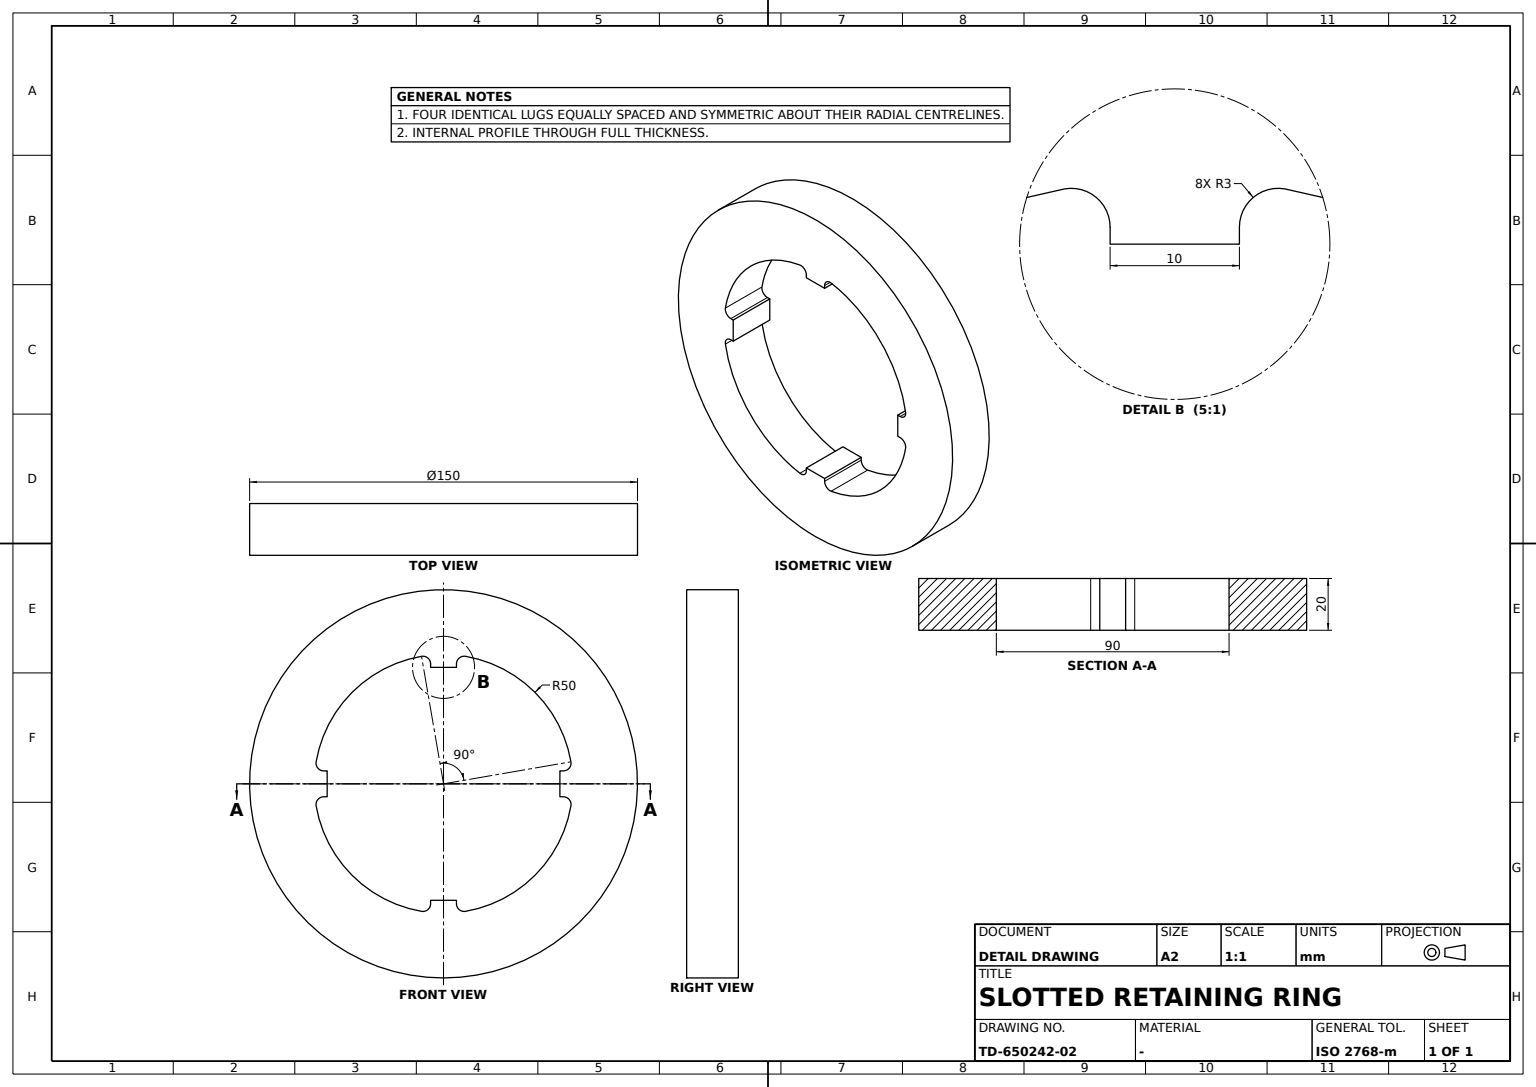
ISO-10303-21;
HEADER;
FILE_DESCRIPTION((''),'2;1');
FILE_NAME('','',(''),(''),'','','');
FILE_SCHEMA(('AUTOMOTIVE_DESIGN'));
ENDSEC;
DATA;
#1=APPLICATION_CONTEXT('');
#2=PRODUCT_CONTEXT('',#1,'mechanical');
#3=PRODUCT('','','',(#2));
#4=PRODUCT_DEFINITION_FORMATION('','',#3);
#5=PRODUCT_DEFINITION_CONTEXT('',#1,'design');
#6=PRODUCT_DEFINITION('','',#4,#5);
#7=PRODUCT_DEFINITION_SHAPE('','',#6);
#8=(LENGTH_UNIT()NAMED_UNIT(*)SI_UNIT(.MILLI.,.METRE.));
#9=(NAMED_UNIT(*)PLANE_ANGLE_UNIT()SI_UNIT($,.RADIAN.));
#10=(NAMED_UNIT(*)SI_UNIT($,.STERADIAN.)SOLID_ANGLE_UNIT());
#11=UNCERTAINTY_MEASURE_WITH_UNIT(LENGTH_MEASURE(0.005),#8,'distance_accuracy_value','');
#12=(GEOMETRIC_REPRESENTATION_CONTEXT(3)GLOBAL_UNCERTAINTY_ASSIGNED_CONTEXT((#11))GLOBAL_UNIT_ASSIGNED_CONTEXT((#8,#9,#10))REPRESENTATION_CONTEXT('',''));
#13=CARTESIAN_POINT('',(-10.,49.270367,8.510638));
#14=VERTEX_POINT('',#13);
#15=CARTESIAN_POINT('',(10.,49.270367,8.510638));
#16=VERTEX_POINT('',#15);
#17=CARTESIAN_POINT('',(0.,49.270367,8.510638));
#18=DIRECTION('',(1.,0.,0.));
#19=VECTOR('',#18,1000.);
#20=LINE('',#17,#19);
#21=EDGE_CURVE('',#14,#16,#20,.T.);
#22=ORIENTED_EDGE('',*,*,#21,.F.);
#23=CARTESIAN_POINT('',(-10.,46.314145,5.));
#24=VERTEX_POINT('',#23);
#25=CARTESIAN_POINT('',(-10.,46.314145,8.));
#26=DIRECTION('',(0.,0.,-1.));
#27=AXIS2_PLACEMENT_3D('',#25,#18,#26);
#28=CIRCLE('',#27,3.);
#29=EDGE_CURVE('',#24,#14,#28,.T.);
#30=ORIENTED_EDGE('',*,*,#29,.F.);
#31=CARTESIAN_POINT('',(10.,46.314145,5.));
#32=VERTEX_POINT('',#31);
#33=CARTESIAN_POINT('',(0.,46.314145,5.));
#34=LINE('',#33,#19);
#35=EDGE_CURVE('',#24,#32,#34,.T.);
#36=ORIENTED_EDGE('',*,*,#35,.T.);
#37=CARTESIAN_POINT('',(10.,46.314145,8.));
#38=AXIS2_PLACEMENT_3D('',#37,#18,#26);
#39=CIRCLE('',#38,3.);
#40=EDGE_CURVE('',#32,#16,#39,.T.);
#41=ORIENTED_EDGE('',*,*,#40,.T.);
#42=EDGE_LOOP('',(#22,#30,#36,#41));
#43=FACE_BOUND('',#42,.T.);
#44=CARTESIAN_POINT('',(0.,46.314145,8.));
#45=DIRECTION('',(0.,1.,0.));
#46=AXIS2_PLACEMENT_3D('',#44,#18,#45);
#47=CYLINDRICAL_SURFACE('',#46,3.);
#48=ADVANCED_FACE('',(#43),#47,.F.);
#49=CARTESIAN_POINT('',(-10.,-46.314145,5.));
#50=VERTEX_POINT('',#49);
#51=CARTESIAN_POINT('',(-10.,-45.,5.));
#52=VERTEX_POINT('',#51);
#53=CARTESIAN_POINT('',(-10.,0.,5.));
#54=VECTOR('',#45,1000.);
#55=LINE('',#53,#54);
#56=EDGE_CURVE('',#50,#52,#55,.T.);
#57=ORIENTED_EDGE('',*,*,#56,.F.);
#58=CARTESIAN_POINT('',(10.,-46.314145,5.));
#59=VERTEX_POINT('',#58);
#60=CARTESIAN_POINT('',(0.,-46.314145,5.));
#61=LINE('',#60,#19);
#62=EDGE_CURVE('',#50,#59,#61,.T.);
#63=ORIENTED_EDGE('',*,*,#62,.T.);
#64=CARTESIAN_POINT('',(10.,-45.,5.));
#65=VERTEX_POINT('',#64);
#66=CARTESIAN_POINT('',(10.,0.,5.));
#67=LINE('',#66,#54);
#68=EDGE_CURVE('',#59,#65,#67,.T.);
#69=ORIENTED_EDGE('',*,*,#68,.T.);
#70=CARTESIAN_POINT('',(0.,-45.,5.));
#71=LINE('',#70,#19);
#72=EDGE_CURVE('',#52,#65,#71,.T.);
#73=ORIENTED_EDGE('',*,*,#72,.F.);
#74=EDGE_LOOP('',(#57,#63,#69,#73));
#75=FACE_BOUND('',#74,.T.);
#76=AXIS2_PLACEMENT_3D('',#60,#26,#45);
#77=PLANE('',#76);
#78=ADVANCED_FACE('',(#75),#77,.F.);
#79=CARTESIAN_POINT('',(10.,45.,5.));
#80=VERTEX_POINT('',#79);
#81=EDGE_CURVE('',#80,#32,#67,.T.);
#82=ORIENTED_EDGE('',*,*,#81,.F.);
#83=CARTESIAN_POINT('',(10.,45.,-5.));
#84=VERTEX_POINT('',#83);
#85=CARTESIAN_POINT('',(10.,45.,0.));
#86=DIRECTION('',(0.,0.,1.));
#87=VECTOR('',#86,1000.);
#88=LINE('',#85,#87);
#89=EDGE_CURVE('',#84,#80,#88,.T.);
#90=ORIENTED_EDGE('',*,*,#89,.F.);
#91=CARTESIAN_POINT('',(10.,46.314145,-5.));
#92=VERTEX_POINT('',#91);
#93=CARTESIAN_POINT('',(10.,0.,-5.));
#94=DIRECTION('',(0.,-1.,0.));
#95=VECTOR('',#94,1000.);
#96=LINE('',#93,#95);
#97=EDGE_CURVE('',#92,#84,#96,.T.);
#98=ORIENTED_EDGE('',*,*,#97,.F.);
#99=CARTESIAN_POINT('',(10.,49.270367,-8.510638));
#100=VERTEX_POINT('',#99);
#101=CARTESIAN_POINT('',(10.,46.314145,-8.));
#102=AXIS2_PLACEMENT_3D('',#101,#18,#26);
#103=CIRCLE('',#102,3.);
#104=EDGE_CURVE('',#100,#92,#103,.T.);
#105=ORIENTED_EDGE('',*,*,#104,.F.);
#106=CARTESIAN_POINT('',(10.,8.510638,-49.270367));
#107=VERTEX_POINT('',#106);
#108=CARTESIAN_POINT('',(10.,0.,0.));
#109=AXIS2_PLACEMENT_3D('',#108,#18,#26);
#110=CIRCLE('',#109,50.);
#111=EDGE_CURVE('',#107,#100,#110,.T.);
#112=ORIENTED_EDGE('',*,*,#111,.F.);
#113=CARTESIAN_POINT('',(10.,5.,-46.314145));
#114=VERTEX_POINT('',#113);
#115=CARTESIAN_POINT('',(10.,8.,-46.314145));
#116=AXIS2_PLACEMENT_3D('',#115,#18,#26);
#117=CIRCLE('',#116,3.);
#118=EDGE_CURVE('',#114,#107,#117,.T.);
#119=ORIENTED_EDGE('',*,*,#118,.F.);
#120=CARTESIAN_POINT('',(10.,5.,-45.));
#121=VERTEX_POINT('',#120);
#122=CARTESIAN_POINT('',(10.,5.,0.));
#123=VECTOR('',#26,1000.);
#124=LINE('',#122,#123);
#125=EDGE_CURVE('',#121,#114,#124,.T.);
#126=ORIENTED_EDGE('',*,*,#125,.F.);
#127=CARTESIAN_POINT('',(10.,-5.,-45.));
#128=VERTEX_POINT('',#127);
#129=CARTESIAN_POINT('',(10.,0.,-45.));
#130=LINE('',#129,#54);
#131=EDGE_CURVE('',#128,#121,#130,.T.);
#132=ORIENTED_EDGE('',*,*,#131,.F.);
#133=CARTESIAN_POINT('',(10.,-5.,-46.314145));
#134=VERTEX_POINT('',#133);
#135=CARTESIAN_POINT('',(10.,-5.,0.));
#136=LINE('',#135,#87);
#137=EDGE_CURVE('',#134,#128,#136,.T.);
#138=ORIENTED_EDGE('',*,*,#137,.F.);
#139=CARTESIAN_POINT('',(10.,-8.510638,-49.270367));
#140=VERTEX_POINT('',#139);
#141=CARTESIAN_POINT('',(10.,-8.,-46.314145));
#142=AXIS2_PLACEMENT_3D('',#141,#18,#26);
#143=CIRCLE('',#142,3.);
#144=EDGE_CURVE('',#140,#134,#143,.T.);
#145=ORIENTED_EDGE('',*,*,#144,.F.);
#146=CARTESIAN_POINT('',(10.,-49.270367,-8.510638));
#147=VERTEX_POINT('',#146);
#148=EDGE_CURVE('',#147,#140,#110,.T.);
#149=ORIENTED_EDGE('',*,*,#148,.F.);
#150=CARTESIAN_POINT('',(10.,-46.314145,-5.));
#151=VERTEX_POINT('',#150);
#152=CARTESIAN_POINT('',(10.,-46.314145,-8.));
#153=AXIS2_PLACEMENT_3D('',#152,#18,#26);
#154=CIRCLE('',#153,3.);
#155=EDGE_CURVE('',#151,#147,#154,.T.);
#156=ORIENTED_EDGE('',*,*,#155,.F.);
#157=CARTESIAN_POINT('',(10.,-45.,-5.));
#158=VERTEX_POINT('',#157);
#159=EDGE_CURVE('',#158,#151,#96,.T.);
#160=ORIENTED_EDGE('',*,*,#159,.F.);
#161=CARTESIAN_POINT('',(10.,-45.,0.));
#162=LINE('',#161,#123);
#163=EDGE_CURVE('',#65,#158,#162,.T.);
#164=ORIENTED_EDGE('',*,*,#163,.F.);
#165=ORIENTED_EDGE('',*,*,#68,.F.);
#166=CARTESIAN_POINT('',(10.,-49.270367,8.510638));
#167=VERTEX_POINT('',#166);
#168=CARTESIAN_POINT('',(10.,-46.314145,8.));
#169=AXIS2_PLACEMENT_3D('',#168,#18,#26);
#170=CIRCLE('',#169,3.);
#171=EDGE_CURVE('',#167,#59,#170,.T.);
#172=ORIENTED_EDGE('',*,*,#171,.F.);
#173=CARTESIAN_POINT('',(10.,-8.510638,49.270367));
#174=VERTEX_POINT('',#173);
#175=EDGE_CURVE('',#174,#167,#110,.T.);
#176=ORIENTED_EDGE('',*,*,#175,.F.);
#177=CARTESIAN_POINT('',(10.,-5.,46.314145));
#178=VERTEX_POINT('',#177);
#179=CARTESIAN_POINT('',(10.,-8.,46.314145));
#180=AXIS2_PLACEMENT_3D('',#179,#18,#26);
#181=CIRCLE('',#180,3.);
#182=EDGE_CURVE('',#178,#174,#181,.T.);
#183=ORIENTED_EDGE('',*,*,#182,.F.);
#184=CARTESIAN_POINT('',(10.,-5.,45.));
#185=VERTEX_POINT('',#184);
#186=EDGE_CURVE('',#185,#178,#136,.T.);
#187=ORIENTED_EDGE('',*,*,#186,.F.);
#188=CARTESIAN_POINT('',(10.,5.,45.));
#189=VERTEX_POINT('',#188);
#190=CARTESIAN_POINT('',(10.,0.,45.));
#191=LINE('',#190,#95);
#192=EDGE_CURVE('',#189,#185,#191,.T.);
#193=ORIENTED_EDGE('',*,*,#192,.F.);
#194=CARTESIAN_POINT('',(10.,5.,46.314145));
#195=VERTEX_POINT('',#194);
#196=EDGE_CURVE('',#195,#189,#124,.T.);
#197=ORIENTED_EDGE('',*,*,#196,.F.);
#198=CARTESIAN_POINT('',(10.,8.510638,49.270367));
#199=VERTEX_POINT('',#198);
#200=CARTESIAN_POINT('',(10.,8.,46.314145));
#201=AXIS2_PLACEMENT_3D('',#200,#18,#26);
#202=CIRCLE('',#201,3.);
#203=EDGE_CURVE('',#199,#195,#202,.T.);
#204=ORIENTED_EDGE('',*,*,#203,.F.);
#205=EDGE_CURVE('',#16,#199,#110,.T.);
#206=ORIENTED_EDGE('',*,*,#205,.F.);
#207=ORIENTED_EDGE('',*,*,#40,.F.);
#208=EDGE_LOOP('',(#82,#90,#98,#105,#112,#119,#126,#132,#138,#145,#149,#156,#160,#164,#165,#172,#176,#183,#187,#193,#197,#204,#206,#207));
#209=FACE_BOUND('',#208,.T.);
#210=CARTESIAN_POINT('',(10.,0.,-75.));
#211=VERTEX_POINT('',#210);
#212=CIRCLE('',#109,75.);
#213=EDGE_CURVE('',#211,#211,#212,.T.);
#214=ORIENTED_EDGE('',*,*,#213,.T.);
#215=EDGE_LOOP('',(#214));
#216=FACE_BOUND('',#215,.T.);
#217=AXIS2_PLACEMENT_3D('',#108,#18,#45);
#218=PLANE('',#217);
#219=ADVANCED_FACE('',(#209,#216),#218,.T.);
#220=CARTESIAN_POINT('',(-10.,-8.510638,49.270367));
#221=VERTEX_POINT('',#220);
#222=CARTESIAN_POINT('',(-10.,-49.270367,8.510638));
#223=VERTEX_POINT('',#222);
#224=CARTESIAN_POINT('',(-10.,0.,0.));
#225=AXIS2_PLACEMENT_3D('',#224,#18,#26);
#226=CIRCLE('',#225,50.);
#227=EDGE_CURVE('',#221,#223,#226,.T.);
#228=ORIENTED_EDGE('',*,*,#227,.F.);
#229=CARTESIAN_POINT('',(0.,-8.510638,49.270367));
#230=LINE('',#229,#19);
#231=EDGE_CURVE('',#221,#174,#230,.T.);
#232=ORIENTED_EDGE('',*,*,#231,.T.);
#233=ORIENTED_EDGE('',*,*,#175,.T.);
#234=CARTESIAN_POINT('',(0.,-49.270367,8.510638));
#235=LINE('',#234,#19);
#236=EDGE_CURVE('',#223,#167,#235,.T.);
#237=ORIENTED_EDGE('',*,*,#236,.F.);
#238=EDGE_LOOP('',(#228,#232,#233,#237));
#239=FACE_BOUND('',#238,.T.);
#240=CARTESIAN_POINT('',(0.,0.,0.));
#241=AXIS2_PLACEMENT_3D('',#240,#18,#45);
#242=CYLINDRICAL_SURFACE('',#241,50.);
#243=ADVANCED_FACE('',(#239),#242,.F.);
#244=CARTESIAN_POINT('',(-10.,8.510638,-49.270367));
#245=VERTEX_POINT('',#244);
#246=CARTESIAN_POINT('',(0.,8.510638,-49.270367));
#247=LINE('',#246,#19);
#248=EDGE_CURVE('',#245,#107,#247,.T.);
#249=ORIENTED_EDGE('',*,*,#248,.T.);
#250=ORIENTED_EDGE('',*,*,#111,.T.);
#251=CARTESIAN_POINT('',(-10.,49.270367,-8.510638));
#252=VERTEX_POINT('',#251);
#253=CARTESIAN_POINT('',(0.,49.270367,-8.510638));
#254=LINE('',#253,#19);
#255=EDGE_CURVE('',#252,#100,#254,.T.);
#256=ORIENTED_EDGE('',*,*,#255,.F.);
#257=EDGE_CURVE('',#245,#252,#226,.T.);
#258=ORIENTED_EDGE('',*,*,#257,.F.);
#259=EDGE_LOOP('',(#249,#250,#256,#258));
#260=FACE_BOUND('',#259,.T.);
#261=ADVANCED_FACE('',(#260),#242,.F.);
#262=CARTESIAN_POINT('',(-10.,5.,46.314145));
#263=VERTEX_POINT('',#262);
#264=CARTESIAN_POINT('',(-10.,5.,45.));
#265=VERTEX_POINT('',#264);
#266=CARTESIAN_POINT('',(-10.,5.,0.));
#267=LINE('',#266,#123);
#268=EDGE_CURVE('',#263,#265,#267,.T.);
#269=ORIENTED_EDGE('',*,*,#268,.F.);
#270=CARTESIAN_POINT('',(0.,5.,46.314145));
#271=LINE('',#270,#19);
#272=EDGE_CURVE('',#263,#195,#271,.T.);
#273=ORIENTED_EDGE('',*,*,#272,.T.);
#274=ORIENTED_EDGE('',*,*,#196,.T.);
#275=CARTESIAN_POINT('',(0.,5.,45.));
#276=LINE('',#275,#19);
#277=EDGE_CURVE('',#265,#189,#276,.T.);
#278=ORIENTED_EDGE('',*,*,#277,.F.);
#279=EDGE_LOOP('',(#269,#273,#274,#278));
#280=FACE_BOUND('',#279,.T.);
#281=CARTESIAN_POINT('',(0.,5.,-45.));
#282=AXIS2_PLACEMENT_3D('',#281,#94,#26);
#283=PLANE('',#282);
#284=ADVANCED_FACE('',(#280),#283,.F.);
#285=ORIENTED_EDGE('',*,*,#125,.T.);
#286=CARTESIAN_POINT('',(-10.,5.,-46.314145));
#287=VERTEX_POINT('',#286);
#288=CARTESIAN_POINT('',(0.,5.,-46.314145));
#289=LINE('',#288,#19);
#290=EDGE_CURVE('',#287,#114,#289,.T.);
#291=ORIENTED_EDGE('',*,*,#290,.F.);
#292=CARTESIAN_POINT('',(-10.,5.,-45.));
#293=VERTEX_POINT('',#292);
#294=EDGE_CURVE('',#293,#287,#267,.T.);
#295=ORIENTED_EDGE('',*,*,#294,.F.);
#296=LINE('',#281,#19);
#297=EDGE_CURVE('',#293,#121,#296,.T.);
#298=ORIENTED_EDGE('',*,*,#297,.T.);
#299=EDGE_LOOP('',(#285,#291,#295,#298));
#300=FACE_BOUND('',#299,.T.);
#301=ADVANCED_FACE('',(#300),#283,.F.);
#302=ORIENTED_EDGE('',*,*,#231,.F.);
#303=CARTESIAN_POINT('',(-10.,-5.,46.314145));
#304=VERTEX_POINT('',#303);
#305=CARTESIAN_POINT('',(-10.,-8.,46.314145));
#306=AXIS2_PLACEMENT_3D('',#305,#18,#26);
#307=CIRCLE('',#306,3.);
#308=EDGE_CURVE('',#304,#221,#307,.T.);
#309=ORIENTED_EDGE('',*,*,#308,.F.);
#310=CARTESIAN_POINT('',(0.,-5.,46.314145));
#311=LINE('',#310,#19);
#312=EDGE_CURVE('',#304,#178,#311,.T.);
#313=ORIENTED_EDGE('',*,*,#312,.T.);
#314=ORIENTED_EDGE('',*,*,#182,.T.);
#315=EDGE_LOOP('',(#302,#309,#313,#314));
#316=FACE_BOUND('',#315,.T.);
#317=CARTESIAN_POINT('',(0.,-8.,46.314145));
#318=AXIS2_PLACEMENT_3D('',#317,#18,#45);
#319=CYLINDRICAL_SURFACE('',#318,3.);
#320=ADVANCED_FACE('',(#316),#319,.F.);
#321=ORIENTED_EDGE('',*,*,#297,.F.);
#322=CARTESIAN_POINT('',(-10.,-5.,-45.));
#323=VERTEX_POINT('',#322);
#324=CARTESIAN_POINT('',(-10.,0.,-45.));
#325=LINE('',#324,#54);
#326=EDGE_CURVE('',#323,#293,#325,.T.);
#327=ORIENTED_EDGE('',*,*,#326,.F.);
#328=CARTESIAN_POINT('',(0.,-5.,-45.));
#329=LINE('',#328,#19);
#330=EDGE_CURVE('',#323,#128,#329,.T.);
#331=ORIENTED_EDGE('',*,*,#330,.T.);
#332=ORIENTED_EDGE('',*,*,#131,.T.);
#333=EDGE_LOOP('',(#321,#327,#331,#332));
#334=FACE_BOUND('',#333,.T.);
#335=AXIS2_PLACEMENT_3D('',#328,#26,#45);
#336=PLANE('',#335);
#337=ADVANCED_FACE('',(#334),#336,.F.);
#338=CARTESIAN_POINT('',(-10.,-8.510638,-49.270367));
#339=VERTEX_POINT('',#338);
#340=CARTESIAN_POINT('',(-10.,-5.,-46.314145));
#341=VERTEX_POINT('',#340);
#342=CARTESIAN_POINT('',(-10.,-8.,-46.314145));
#343=AXIS2_PLACEMENT_3D('',#342,#18,#26);
#344=CIRCLE('',#343,3.);
#345=EDGE_CURVE('',#339,#341,#344,.T.);
#346=ORIENTED_EDGE('',*,*,#345,.T.);
#347=CARTESIAN_POINT('',(-10.,-5.,0.));
#348=LINE('',#347,#87);
#349=EDGE_CURVE('',#341,#323,#348,.T.);
#350=ORIENTED_EDGE('',*,*,#349,.T.);
#351=ORIENTED_EDGE('',*,*,#326,.T.);
#352=ORIENTED_EDGE('',*,*,#294,.T.);
#353=CARTESIAN_POINT('',(-10.,8.,-46.314145));
#354=AXIS2_PLACEMENT_3D('',#353,#18,#26);
#355=CIRCLE('',#354,3.);
#356=EDGE_CURVE('',#287,#245,#355,.T.);
#357=ORIENTED_EDGE('',*,*,#356,.T.);
#358=ORIENTED_EDGE('',*,*,#257,.T.);
#359=CARTESIAN_POINT('',(-10.,46.314145,-5.));
#360=VERTEX_POINT('',#359);
#361=CARTESIAN_POINT('',(-10.,46.314145,-8.));
#362=AXIS2_PLACEMENT_3D('',#361,#18,#26);
#363=CIRCLE('',#362,3.);
#364=EDGE_CURVE('',#252,#360,#363,.T.);
#365=ORIENTED_EDGE('',*,*,#364,.T.);
#366=CARTESIAN_POINT('',(-10.,45.,-5.));
#367=VERTEX_POINT('',#366);
#368=CARTESIAN_POINT('',(-10.,0.,-5.));
#369=LINE('',#368,#95);
#370=EDGE_CURVE('',#360,#367,#369,.T.);
#371=ORIENTED_EDGE('',*,*,#370,.T.);
#372=CARTESIAN_POINT('',(-10.,45.,5.));
#373=VERTEX_POINT('',#372);
#374=CARTESIAN_POINT('',(-10.,45.,0.));
#375=LINE('',#374,#87);
#376=EDGE_CURVE('',#367,#373,#375,.T.);
#377=ORIENTED_EDGE('',*,*,#376,.T.);
#378=EDGE_CURVE('',#373,#24,#55,.T.);
#379=ORIENTED_EDGE('',*,*,#378,.T.);
#380=ORIENTED_EDGE('',*,*,#29,.T.);
#381=CARTESIAN_POINT('',(-10.,8.510638,49.270367));
#382=VERTEX_POINT('',#381);
#383=EDGE_CURVE('',#14,#382,#226,.T.);
#384=ORIENTED_EDGE('',*,*,#383,.T.);
#385=CARTESIAN_POINT('',(-10.,8.,46.314145));
#386=AXIS2_PLACEMENT_3D('',#385,#18,#26);
#387=CIRCLE('',#386,3.);
#388=EDGE_CURVE('',#382,#263,#387,.T.);
#389=ORIENTED_EDGE('',*,*,#388,.T.);
#390=ORIENTED_EDGE('',*,*,#268,.T.);
#391=CARTESIAN_POINT('',(-10.,-5.,45.));
#392=VERTEX_POINT('',#391);
#393=CARTESIAN_POINT('',(-10.,0.,45.));
#394=LINE('',#393,#95);
#395=EDGE_CURVE('',#265,#392,#394,.T.);
#396=ORIENTED_EDGE('',*,*,#395,.T.);
#397=EDGE_CURVE('',#392,#304,#348,.T.);
#398=ORIENTED_EDGE('',*,*,#397,.T.);
#399=ORIENTED_EDGE('',*,*,#308,.T.);
#400=ORIENTED_EDGE('',*,*,#227,.T.);
#401=CARTESIAN_POINT('',(-10.,-46.314145,8.));
#402=AXIS2_PLACEMENT_3D('',#401,#18,#26);
#403=CIRCLE('',#402,3.);
#404=EDGE_CURVE('',#223,#50,#403,.T.);
#405=ORIENTED_EDGE('',*,*,#404,.T.);
#406=ORIENTED_EDGE('',*,*,#56,.T.);
#407=CARTESIAN_POINT('',(-10.,-45.,-5.));
#408=VERTEX_POINT('',#407);
#409=CARTESIAN_POINT('',(-10.,-45.,0.));
#410=LINE('',#409,#123);
#411=EDGE_CURVE('',#52,#408,#410,.T.);
#412=ORIENTED_EDGE('',*,*,#411,.T.);
#413=CARTESIAN_POINT('',(-10.,-46.314145,-5.));
#414=VERTEX_POINT('',#413);
#415=EDGE_CURVE('',#408,#414,#369,.T.);
#416=ORIENTED_EDGE('',*,*,#415,.T.);
#417=CARTESIAN_POINT('',(-10.,-49.270367,-8.510638));
#418=VERTEX_POINT('',#417);
#419=CARTESIAN_POINT('',(-10.,-46.314145,-8.));
#420=AXIS2_PLACEMENT_3D('',#419,#18,#26);
#421=CIRCLE('',#420,3.);
#422=EDGE_CURVE('',#414,#418,#421,.T.);
#423=ORIENTED_EDGE('',*,*,#422,.T.);
#424=EDGE_CURVE('',#418,#339,#226,.T.);
#425=ORIENTED_EDGE('',*,*,#424,.T.);
#426=EDGE_LOOP('',(#346,#350,#351,#352,#357,#358,#365,#371,#377,#379,#380,#384,#389,#390,#396,#398,#399,#400,#405,#406,#412,#416,#423,#425));
#427=FACE_BOUND('',#426,.T.);
#428=CARTESIAN_POINT('',(-10.,0.,-75.));
#429=VERTEX_POINT('',#428);
#430=CIRCLE('',#225,75.);
#431=EDGE_CURVE('',#429,#429,#430,.T.);
#432=ORIENTED_EDGE('',*,*,#431,.F.);
#433=EDGE_LOOP('',(#432));
#434=FACE_BOUND('',#433,.T.);
#435=AXIS2_PLACEMENT_3D('',#224,#18,#45);
#436=PLANE('',#435);
#437=ADVANCED_FACE('',(#427,#434),#436,.F.);
#438=ORIENTED_EDGE('',*,*,#186,.T.);
#439=ORIENTED_EDGE('',*,*,#312,.F.);
#440=ORIENTED_EDGE('',*,*,#397,.F.);
#441=CARTESIAN_POINT('',(0.,-5.,45.));
#442=LINE('',#441,#19);
#443=EDGE_CURVE('',#392,#185,#442,.T.);
#444=ORIENTED_EDGE('',*,*,#443,.T.);
#445=EDGE_LOOP('',(#438,#439,#440,#444));
#446=FACE_BOUND('',#445,.T.);
#447=CARTESIAN_POINT('',(0.,-5.,-46.314145));
#448=AXIS2_PLACEMENT_3D('',#447,#45,#86);
#449=PLANE('',#448);
#450=ADVANCED_FACE('',(#446),#449,.F.);
#451=CARTESIAN_POINT('',(0.,-46.314145,-5.));
#452=LINE('',#451,#19);
#453=EDGE_CURVE('',#414,#151,#452,.T.);
#454=ORIENTED_EDGE('',*,*,#453,.F.);
#455=ORIENTED_EDGE('',*,*,#415,.F.);
#456=CARTESIAN_POINT('',(0.,-45.,-5.));
#457=LINE('',#456,#19);
#458=EDGE_CURVE('',#408,#158,#457,.T.);
#459=ORIENTED_EDGE('',*,*,#458,.T.);
#460=ORIENTED_EDGE('',*,*,#159,.T.);
#461=EDGE_LOOP('',(#454,#455,#459,#460));
#462=FACE_BOUND('',#461,.T.);
#463=AXIS2_PLACEMENT_3D('',#456,#86,#94);
#464=PLANE('',#463);
#465=ADVANCED_FACE('',(#462),#464,.F.);
#466=ORIENTED_EDGE('',*,*,#171,.T.);
#467=ORIENTED_EDGE('',*,*,#62,.F.);
#468=ORIENTED_EDGE('',*,*,#404,.F.);
#469=ORIENTED_EDGE('',*,*,#236,.T.);
#470=EDGE_LOOP('',(#466,#467,#468,#469));
#471=FACE_BOUND('',#470,.T.);
#472=CARTESIAN_POINT('',(0.,-46.314145,8.));
#473=AXIS2_PLACEMENT_3D('',#472,#18,#45);
#474=CYLINDRICAL_SURFACE('',#473,3.);
#475=ADVANCED_FACE('',(#471),#474,.F.);
#476=ORIENTED_EDGE('',*,*,#205,.T.);
#477=CARTESIAN_POINT('',(0.,8.510638,49.270367));
#478=LINE('',#477,#19);
#479=EDGE_CURVE('',#382,#199,#478,.T.);
#480=ORIENTED_EDGE('',*,*,#479,.F.);
#481=ORIENTED_EDGE('',*,*,#383,.F.);
#482=ORIENTED_EDGE('',*,*,#21,.T.);
#483=EDGE_LOOP('',(#476,#480,#481,#482));
#484=FACE_BOUND('',#483,.T.);
#485=ADVANCED_FACE('',(#484),#242,.F.);
#486=ORIENTED_EDGE('',*,*,#458,.F.);
#487=ORIENTED_EDGE('',*,*,#411,.F.);
#488=ORIENTED_EDGE('',*,*,#72,.T.);
#489=ORIENTED_EDGE('',*,*,#163,.T.);
#490=EDGE_LOOP('',(#486,#487,#488,#489));
#491=FACE_BOUND('',#490,.T.);
#492=AXIS2_PLACEMENT_3D('',#70,#94,#26);
#493=PLANE('',#492);
#494=ADVANCED_FACE('',(#491),#493,.F.);
#495=CARTESIAN_POINT('',(0.,46.314145,-5.));
#496=LINE('',#495,#19);
#497=EDGE_CURVE('',#360,#92,#496,.T.);
#498=ORIENTED_EDGE('',*,*,#497,.T.);
#499=ORIENTED_EDGE('',*,*,#97,.T.);
#500=CARTESIAN_POINT('',(0.,45.,-5.));
#501=LINE('',#500,#19);
#502=EDGE_CURVE('',#367,#84,#501,.T.);
#503=ORIENTED_EDGE('',*,*,#502,.F.);
#504=ORIENTED_EDGE('',*,*,#370,.F.);
#505=EDGE_LOOP('',(#498,#499,#503,#504));
#506=FACE_BOUND('',#505,.T.);
#507=ADVANCED_FACE('',(#506),#464,.F.);
#508=ORIENTED_EDGE('',*,*,#118,.T.);
#509=ORIENTED_EDGE('',*,*,#248,.F.);
#510=ORIENTED_EDGE('',*,*,#356,.F.);
#511=ORIENTED_EDGE('',*,*,#290,.T.);
#512=EDGE_LOOP('',(#508,#509,#510,#511));
#513=FACE_BOUND('',#512,.T.);
#514=CARTESIAN_POINT('',(0.,8.,-46.314145));
#515=AXIS2_PLACEMENT_3D('',#514,#18,#45);
#516=CYLINDRICAL_SURFACE('',#515,3.);
#517=ADVANCED_FACE('',(#513),#516,.F.);
#518=ORIENTED_EDGE('',*,*,#277,.T.);
#519=ORIENTED_EDGE('',*,*,#192,.T.);
#520=ORIENTED_EDGE('',*,*,#443,.F.);
#521=ORIENTED_EDGE('',*,*,#395,.F.);
#522=EDGE_LOOP('',(#518,#519,#520,#521));
#523=FACE_BOUND('',#522,.T.);
#524=AXIS2_PLACEMENT_3D('',#275,#86,#94);
#525=PLANE('',#524);
#526=ADVANCED_FACE('',(#523),#525,.F.);
#527=ORIENTED_EDGE('',*,*,#388,.F.);
#528=ORIENTED_EDGE('',*,*,#479,.T.);
#529=ORIENTED_EDGE('',*,*,#203,.T.);
#530=ORIENTED_EDGE('',*,*,#272,.F.);
#531=EDGE_LOOP('',(#527,#528,#529,#530));
#532=FACE_BOUND('',#531,.T.);
#533=CARTESIAN_POINT('',(0.,8.,46.314145));
#534=AXIS2_PLACEMENT_3D('',#533,#18,#45);
#535=CYLINDRICAL_SURFACE('',#534,3.);
#536=ADVANCED_FACE('',(#532),#535,.F.);
#537=ORIENTED_EDGE('',*,*,#148,.T.);
#538=CARTESIAN_POINT('',(0.,-8.510638,-49.270367));
#539=LINE('',#538,#19);
#540=EDGE_CURVE('',#339,#140,#539,.T.);
#541=ORIENTED_EDGE('',*,*,#540,.F.);
#542=ORIENTED_EDGE('',*,*,#424,.F.);
#543=CARTESIAN_POINT('',(0.,-49.270367,-8.510638));
#544=LINE('',#543,#19);
#545=EDGE_CURVE('',#418,#147,#544,.T.);
#546=ORIENTED_EDGE('',*,*,#545,.T.);
#547=EDGE_LOOP('',(#537,#541,#542,#546));
#548=FACE_BOUND('',#547,.T.);
#549=ADVANCED_FACE('',(#548),#242,.F.);
#550=ORIENTED_EDGE('',*,*,#349,.F.);
#551=LINE('',#447,#19);
#552=EDGE_CURVE('',#341,#134,#551,.T.);
#553=ORIENTED_EDGE('',*,*,#552,.T.);
#554=ORIENTED_EDGE('',*,*,#137,.T.);
#555=ORIENTED_EDGE('',*,*,#330,.F.);
#556=EDGE_LOOP('',(#550,#553,#554,#555));
#557=FACE_BOUND('',#556,.T.);
#558=ADVANCED_FACE('',(#557),#449,.F.);
#559=ORIENTED_EDGE('',*,*,#453,.T.);
#560=ORIENTED_EDGE('',*,*,#155,.T.);
#561=ORIENTED_EDGE('',*,*,#545,.F.);
#562=ORIENTED_EDGE('',*,*,#422,.F.);
#563=EDGE_LOOP('',(#559,#560,#561,#562));
#564=FACE_BOUND('',#563,.T.);
#565=CARTESIAN_POINT('',(0.,-46.314145,-8.));
#566=AXIS2_PLACEMENT_3D('',#565,#18,#45);
#567=CYLINDRICAL_SURFACE('',#566,3.);
#568=ADVANCED_FACE('',(#564),#567,.F.);
#569=ORIENTED_EDGE('',*,*,#431,.T.);
#570=EDGE_LOOP('',(#569));
#571=FACE_BOUND('',#570,.T.);
#572=ORIENTED_EDGE('',*,*,#213,.F.);
#573=EDGE_LOOP('',(#572));
#574=FACE_BOUND('',#573,.T.);
#575=CYLINDRICAL_SURFACE('',#241,75.);
#576=ADVANCED_FACE('',(#571,#574),#575,.T.);
#577=ORIENTED_EDGE('',*,*,#104,.T.);
#578=ORIENTED_EDGE('',*,*,#497,.F.);
#579=ORIENTED_EDGE('',*,*,#364,.F.);
#580=ORIENTED_EDGE('',*,*,#255,.T.);
#581=EDGE_LOOP('',(#577,#578,#579,#580));
#582=FACE_BOUND('',#581,.T.);
#583=CARTESIAN_POINT('',(0.,46.314145,-8.));
#584=AXIS2_PLACEMENT_3D('',#583,#18,#45);
#585=CYLINDRICAL_SURFACE('',#584,3.);
#586=ADVANCED_FACE('',(#582),#585,.F.);
#587=ORIENTED_EDGE('',*,*,#144,.T.);
#588=ORIENTED_EDGE('',*,*,#552,.F.);
#589=ORIENTED_EDGE('',*,*,#345,.F.);
#590=ORIENTED_EDGE('',*,*,#540,.T.);
#591=EDGE_LOOP('',(#587,#588,#589,#590));
#592=FACE_BOUND('',#591,.T.);
#593=CARTESIAN_POINT('',(0.,-8.,-46.314145));
#594=AXIS2_PLACEMENT_3D('',#593,#18,#45);
#595=CYLINDRICAL_SURFACE('',#594,3.);
#596=ADVANCED_FACE('',(#592),#595,.F.);
#597=ORIENTED_EDGE('',*,*,#35,.F.);
#598=ORIENTED_EDGE('',*,*,#378,.F.);
#599=CARTESIAN_POINT('',(0.,45.,5.));
#600=LINE('',#599,#19);
#601=EDGE_CURVE('',#373,#80,#600,.T.);
#602=ORIENTED_EDGE('',*,*,#601,.T.);
#603=ORIENTED_EDGE('',*,*,#81,.T.);
#604=EDGE_LOOP('',(#597,#598,#602,#603));
#605=FACE_BOUND('',#604,.T.);
#606=ADVANCED_FACE('',(#605),#77,.F.);
#607=ORIENTED_EDGE('',*,*,#376,.F.);
#608=ORIENTED_EDGE('',*,*,#502,.T.);
#609=ORIENTED_EDGE('',*,*,#89,.T.);
#610=ORIENTED_EDGE('',*,*,#601,.F.);
#611=EDGE_LOOP('',(#607,#608,#609,#610));
#612=FACE_BOUND('',#611,.T.);
#613=AXIS2_PLACEMENT_3D('',#500,#45,#86);
#614=PLANE('',#613);
#615=ADVANCED_FACE('',(#612),#614,.F.);
#616=CLOSED_SHELL('',(#48,#78,#219,#243,#261,#284,#301,#320,#337,#437,#450,#465,#475,#485,#494,#507,#517,#526,#536,#549,#558,#568,#576,#586,#596,#606,#615));
#617=MANIFOLD_SOLID_BREP('',#616);
#618=ADVANCED_BREP_SHAPE_REPRESENTATION('',(#617),#12);
#619=SHAPE_DEFINITION_REPRESENTATION(#7,#618);
ENDSEC;
END-ISO-10303-21;
